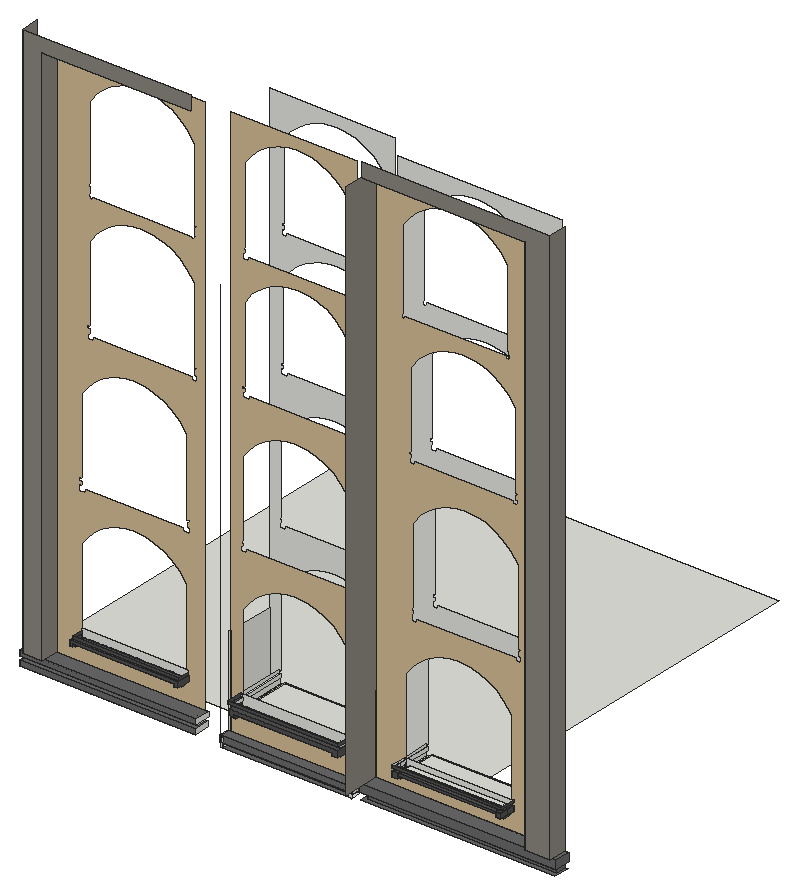
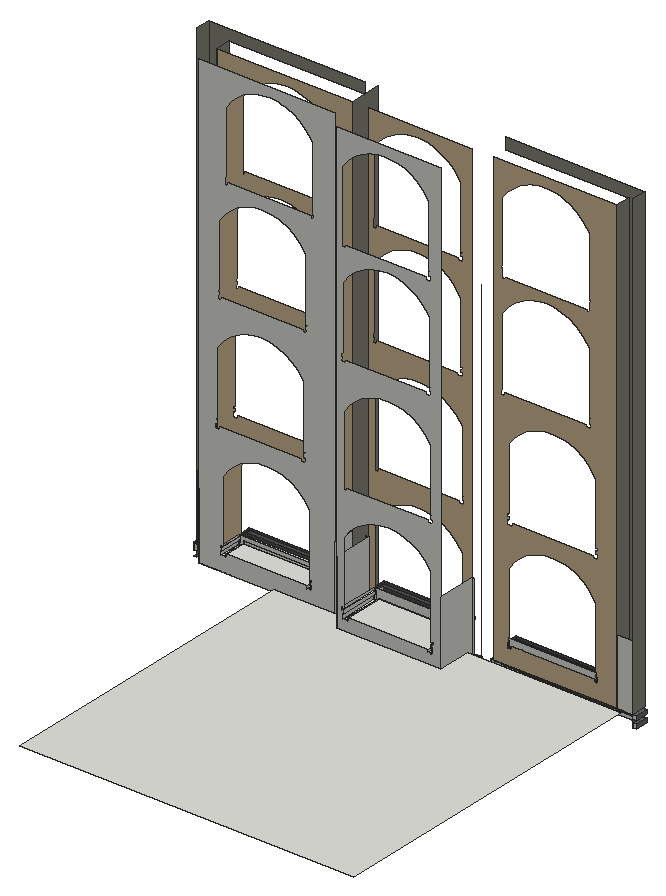
# SketchUp Ruby script. Lengths in inches.
U = 1.inch
M = Sketchup.active_model
def pt(a) = Geom::Point3d.new(a.map { |v| v * U })
def face(e, loops, mat)
  f = e.add_face(loops[0].map { |a| pt(a) })
  loops[1..].each { |l| e.add_face(l.map { |a| pt(a) }).erase! }
  f.material = f.back_material = mat if mat
  f
end
# faces: each face lists its corners as indices into pts; further lists are holes
def faces(e, pts, list, mat = nil) = list.each { |f| face(e, (f[0].is_a?(Array) ? f : [f]).map { |l| l.map { |i| pts[i] } }, mat) }
# xy, xz, yz: faces in a plane at the given z, y or x. An outline is a flat list of corners, or four numbers for a rectangle; further outlines are holes
def ring(l) = l.size == 4 ? [[l[0], l[1]], [l[2], l[1]], [l[2], l[3]], [l[0], l[3]]] : l.each_slice(2).to_a
def flat(e, list, mat, &to3) = list.each { |f| face(e, (f[0].is_a?(Array) ? f : [f]).map { |l| ring(l).map { |u, v| to3.(u, v) } }, mat) }
def xy(e, z, list, mat = nil) = flat(e, list, mat) { |x, y| [x, y, z] }
def xz(e, y, list, mat = nil) = flat(e, list, mat) { |x, z| [x, y, z] }
def yz(e, x, list, mat = nil) = flat(e, list, mat) { |y, z| [x, y, z] }
def lines(e, pts, list) = list.each { |a, b| e.add_line(pt(pts[a]), pt(pts[b])) }
# prism: a flat outline (further loops are holes) pulled along v
def prism(e, loops, v, mat = nil)
  f = face(e, loops, mat); d = Geom::Vector3d.new(v.map { |x| x * U })
  f.pushpull(f.normal.samedirection?(d) ? d.length : -d.length)
end
def box(e, o, s, mat = nil) = prism(e, [[o, [o[0] + s[0], o[1], o[2]], [o[0] + s[0], o[1] + s[1], o[2]], [o[0], o[1] + s[1], o[2]]]], [0, 0, s[2]], mat)
def at(x, y, z, deg = 0) = Geom::Transformation.translation(pt([x, y, z])) * Geom::Transformation.rotation(ORIGIN, Z_AXIS, deg.degrees)
def axes(o, x, y, z) = Geom::Transformation.new([*x, 0, *y, 0, *z, 0, *pt(o).to_a, 1])
def part(name) = M.definitions.add(name)
# library, detail: a bought-in or finely detailed component or shape, given as its bounding box
def library(name, o, s) = part(name).tap { |d| box(d.entities, o, s) }
def detail(e, o, s) = box(e.add_group.entities, o, s)
def put(e, d, t, mat = nil) = e.add_instance(d, t).tap { |i| i.material = mat if mat }
def group(e, t, mat = nil) = e.add_group.tap { |g| g.transformation = t; g.material = mat if mat }.entities
root = M.entities
M.materials.add("[0134_DimGray]").color = [105, 105, 105]
M.materials.add("[0135_DarkGray]").color = [81, 81, 81]
M.materials.add("[Formica Beige]").color = [211, 187, 149]
M.materials.add("[Formica Graystone]").color = [137, 134, 124]
M.materials.add("[Formica Graystone]1").color = [149, 146, 135]
xy(root,125.87,[[224.47,37.6875,226.6,49.6875],[226.6,37.6875,227.04,43.6875],[370.55,37.6875,370.74,43.6875],[370.74,37.6875,374.55,49.6875],[226.6,43.6875,227.04,49.6875],
  [370.55,43.6875,370.74,49.6875],[224.47,49.6875,226.6,107.5]])
xy(root,125.87,[[227.04,37.6875,370.55,43.6875]],"[0134_DimGray]")
xy(root,130.6875,[[223.66,37.6875,223.66,49.6875,226.6,49.6875,226.6,43.6875,370.74,43.6875,370.74,49.6875,375.3,49.6875,375.3,37.6875]],"[0134_DimGray]")
xy(root,131.98,[[389.32,31.6875,611.75,31.6875,611.75,49.6875,608.5,49.6875,608.5,37.6875,392.7,37.6875,392.7,49.6875,389.32,49.6875]],"[0134_DimGray]")
xy(root,132.82,[[0,31.6875,0,49.6875,4.9375,49.6875,4.9375,37.6875,197.35,37.6875,197.35,49.6875,200.6,49.6875,200.6,31.6875]],"[0134_DimGray]")
xy(root,137.74,[[227.04,49.6875,370.55,104.375]])
xy(root,137.74,[[223.66,37.6875,375.3,49.6875]],"[0134_DimGray]")
xy(root,138.5625,[[0,31.6875,200.6,31.6875,200.6,49.6875,197.35,49.6875,197.35,37.6875,4.9375,37.6875,4.9375,49.6875,0,49.6875]],"[0134_DimGray]")
xy(root,139.38,[[387.45,31.6875,387.45,49.6875,392.7,49.6875,392.7,37.6875,608.5,37.6875,608.5,49.6875,612.75,49.6875,612.75,31.6875]],"[0134_DimGray]")
xy(root,143.01,[[0,31.6875,0,49.6875,4.9375,49.6875,4.9375,37.6875,197.35,37.6875,197.35,49.6875,200.97,49.6875,200.97,31.6875]],"[0134_DimGray]")
xy(root,148.75,[[4.9375,31.6875,27.68,49.6875],[387.45,31.6875,392.7,49.6875],[392.7,49.6875,475.9375,80.4375],[475.9375,49.6875,580.01,80.4375]])
xy(root,148.75,[[4.9375,28.6875,27.68,31.6875],[0,31.6875,4.9375,49.6875],[27.68,31.6875,200.97,49.6875],[392.7,31.6875,580.01,49.6875],[580.01,31.6875,612.75,49.6875]],"[0134_DimGray]")
xy(root,149.0625,[[580.01,28.6875,608.5,49.6875]],"[Formica Graystone]1")
xy(root,151.875,[[13.9375,58.6875,475.9375,520.6875]])
xy(root,163.35,[[238.57,34.7,244.63,40.6875]],"[0135_DarkGray]")
xy(root,164.72,[[356.01,37.12,362.82,42.6]],"[0135_DarkGray]")
xy(root,165.85,[[238.57,49.6875,240.45,104.375],[240.45,49.6875,244.63,104.375],[356.01,49.6875,360.89,104.375],[360.89,49.6875,362.82,104.375]])
xy(root,165.85,[[238.57,31.6875,244.63,34.7],[356.01,31.6875,362.82,37.12],[238.57,40.6875,244.63,49.6875],[356.01,42.6,362.82,49.6875]],"[0135_DarkGray]")
xy(root,166.35,[[425.07,35.9375,431.66,40.6875]],"[0135_DarkGray]")
xy(root,167.35,[[543.375,36.53,549.7,42.4375]],"[0135_DarkGray]")
xy(root,168.72,[[425.07,35.9375,426.95,40.6875],[426.95,35.9375,431.66,40.6875],[543.375,36.53,548.14,40.6875],[548.14,36.53,549.7,40.6875],[543.375,40.6875,548.14,42.4375],
  [548.14,40.6875,549.7,42.4375],[425.07,49.6875,426.95,80.4375],[426.95,49.6875,431.66,80.4375],[543.375,49.6875,548.14,80.4375],[548.14,49.6875,549.7,80.4375]])
xy(root,168.72,[[425.07,31.6875,426.95,35.9375],[426.95,31.6875,431.66,35.9375],[543.375,31.6875,548.14,36.53],[548.14,31.6875,549.7,36.53],[425.07,40.6875,426.95,49.6875],
  [426.95,40.6875,431.66,49.6875],[543.375,42.4375,548.14,49.6875],[548.14,42.4375,549.7,49.6875]],"[0135_DarkGray]")
xy(root,168.85,[[244.63,49.6875,356.01,104.375]])
xy(root,168.85,[[244.63,31.6875,356.01,49.6875]],"[0135_DarkGray]")
xy(root,169.47,[[54.45,39.33,58.06,43.45]],"[0135_DarkGray]")
xy(root,169.78,[[173.8125,39.99,177.95,43.12]],"[0135_DarkGray]")
xy(root,171.22,[[54.45,34.6875,58.06,39.33],[173.8125,34.6875,177.95,39.99],[173.8125,43.12,177.95,49.6875],[54.45,43.45,58.06,49.6875]],"[0135_DarkGray]")
xy(root,171.72,[[431.66,49.6875,543.375,80.4375]])
xy(root,171.72,[[431.66,31.6875,543.375,49.6875]],"[0135_DarkGray]")
xy(root,172.92,[[238.57,49.6875,240.45,104.375],[360.89,49.6875,362.82,104.375]])
xy(root,172.92,[[238.57,31.6875,362.82,31.6875,362.82,49.6875,360.89,49.6875,360.89,37.6875,240.45,37.6875,240.45,49.6875,238.57,49.6875]],"[0135_DarkGray]")
xy(root,174.22,[[58.06,34.6875,173.8125,49.6875]],"[0135_DarkGray]")
xy(root,174.33,[[431.66,37.6875,543.375,49.6875],[425.07,49.6875,426.95,80.4375],[548.14,49.6875,549.7,80.4375]])
xy(root,174.33,[[425.07,31.6875,426.95,40.6875],[426.95,31.6875,431.66,37.6875],[431.66,31.6875,543.375,37.6875],[543.375,31.6875,548.14,37.6875],[548.14,31.6875,549.7,40.6875],
  [425.07,40.6875,426.95,49.6875],[548.14,40.6875,549.7,49.6875]],"[0135_DarkGray]")
xy(root,176.99,[[237.76,49.6875,240.45,104.375],[360.89,49.6875,363.26,104.375]])
xy(root,176.99,[[237.76,31.6875,237.76,49.6875,240.45,49.6875,240.45,37.6875,360.89,37.6875,360.89,49.6875,363.26,49.6875,363.26,31.6875]],"[0135_DarkGray]")
xy(root,177.23,[[54.45,34.6875,177.95,34.6875,177.95,49.6875,176.89,49.6875,176.89,37.6875,55.95,37.6875,55.95,49.6875,54.45,49.6875]],"[0135_DarkGray]")
xy(root,178.09,[[425.2,40.6875,426.95,49.6875],[425.2,49.6875,426.95,80.4375],[548.14,49.6875,549.95,80.4375]])
xy(root,178.09,[[425.2,31.6875,426.95,40.6875],[426.95,31.6875,548.14,37.6875],[548.14,31.6875,549.95,40.6875],[548.14,40.6875,549.95,49.6875]],"[0135_DarkGray]")
xz(root,28.6875,[[4.9375,148.75,27.68,148.75,27.68,772.09,197.35,772.09,197.35,787.6875,4.9375,787.6875],[580.01,149.0625,608.5,149.0625,608.5,787.6875,392.7,787.6875,392.7,772.09,580.01,772.09]],"[Formica Graystone]")
xz(root,31.6875,[[0,132.82,200.6,138.5625],[387.45,139.38,612.75,148.75],[0,143.01,200.97,148.75]],"[0134_DimGray]")
xz(root,31.6875,[[238.57,165.85,244.63,165.85,244.63,168.85,356.01,168.85,356.01,165.85,362.82,165.85,362.82,172.92,238.57,172.92],[425.07,168.72,431.66,174.33],[543.375,168.72,549.7,174.33],[431.66,171.72,543.375,174.33],[237.76,176.99,363.26,180.28],
  [425.2,178.09,549.95,180.28]],"[0135_DarkGray]")
xz(root,34.6875,[[54.45,171.22,58.06,171.22,58.06,174.22,173.8125,174.22,173.8125,171.22,177.95,171.22,177.95,177.23,54.45,177.23]],"[0135_DarkGray]")
xz(root,34.7,[[238.57,163.35,244.63,165.85]],"[0135_DarkGray]")
xz(root,35.9375,[[425.07,166.35,431.66,168.72]],"[0135_DarkGray]")
xz(root,36.53,[[543.375,167.35,549.7,168.72]],"[0135_DarkGray]")
xz(root,37.12,[[356.01,164.72,362.82,165.85]],"[0135_DarkGray]")
xz(root,37.6875,[[224.47,125.87,226.6,130.6875],[226.6,125.87,227.04,130.6875],[370.74,125.87,374.55,130.6875],[223.66,130.6875,224.47,137.74],[224.47,130.6875,226.6,137.74],
  [226.6,130.6875,227.04,137.74],[370.55,130.6875,370.74,137.74],[370.74,130.6875,374.55,137.74],[374.55,130.6875,375.3,137.74],[4.9375,132.82,197.35,138.5625]])
xz(root,37.6875,[[227.04,130.6875,370.55,137.74],[392.7,131.98,608.5,139.38],[4.9375,138.5625,197.35,143.01]],"[0134_DimGray]")
xz(root,37.6875,[[240.45,172.92,360.89,176.99],[426.95,174.33,548.14,178.09],[55.95,177.23,176.89,180.23]],"[0135_DarkGray]")
xz(root,39.33,[[54.45,169.47,58.06,171.22]],"[0135_DarkGray]")
xz(root,39.99,[[173.8125,169.78,177.95,171.22]],"[0135_DarkGray]")
xz(root,40.6875,[[238.57,163.35,244.63,165.85],[425.07,166.35,431.66,168.72]])
xz(root,42.4375,[[543.375,167.35,549.7,168.72]])
xz(root,42.6,[[356.01,164.72,362.82,165.85]])
xz(root,43.12,[[173.8125,169.78,177.95,171.22]])
xz(root,43.45,[[54.45,169.47,58.06,171.22]])
xz(root,43.6875,[[226.6,125.87,370.74,130.6875]],"[0134_DimGray]")
xz(root,49.6875,[[224.47,125.87,226.6,130.6875],[226.6,125.87,227.04,130.6875],[370.55,125.87,370.74,130.6875],[370.74,125.87,374.55,130.6875],[223.66,130.6875,224.47,137.74],
  [224.47,130.6875,226.6,137.74],[226.6,130.6875,227.04,137.74],[370.55,130.6875,370.74,137.74],[370.74,130.6875,374.55,137.74],[374.55,130.6875,375.3,137.74],
  [0,132.82,4.9375,138.5625],[197.35,132.82,200.6,138.5625],[224.47,137.74,226.6,240],[226.6,137.74,227.04,240],[370.55,137.74,370.74,240],
  [370.74,137.74,374.55,240],[387.45,139.38,392.7,148.75],[608.5,139.38,612.75,148.75],[0,143.01,4.9375,148.75],[197.35,143.01,200.97,148.75],
  [4.9375,148.75,27.68,240],[580.01,148.75,608.5,149.0625],[580.01,149.0625,608.5,240],[238.57,165.85,240.45,172.92],[240.45,165.85,244.63,165.85,244.63,168.85,356.01,168.85,356.01,165.85,360.89,165.85,360.89,180.28,240.45,180.28],
  [360.89,165.85,362.82,172.92],[425.07,168.72,426.95,174.33],[426.95,168.72,426.95,180.28,548.14,180.28,548.14,168.72,543.375,168.72,543.375,174.33,431.66,174.33,431.66,168.72],[548.14,168.72,549.7,174.33],[54.45,171.22,55.95,177.23],
  [55.95,171.22,58.06,171.22,58.06,174.22,173.8125,174.22,173.8125,171.22,176.89,171.22,176.89,183.1,55.95,183.1],[176.89,171.22,177.95,177.23],[431.66,171.72,543.375,174.33]])
xz(root,49.6875,[[[227.04,137.74,370.55,772.09],[238.57,165.85,238.57,172.92,240.45,172.92,240.45,176.99,237.76,176.99,237.76,180.28,240.45,180.28,240.45,266.7,249.375,278.3,257.84,286.17,267.5,292.53,278.07,297.2,289.27,300.05,300.79,301.01,312.3125,300.05,323.51,297.2,334.09,292.53,343.74,286.17,352.21,278.3,361.14,266.7,361.14,180.28,363.26,180.28,363.26,176.99,360.89,176.99,360.89,172.92,362.82,172.92,362.82,165.85,356.01,165.85,356.01,168.85,244.63,168.85,244.63,165.85],[240.7,626.53,240.7,633.11,242.82,633.11,242.82,636.68,240.7,636.68,240.7,638.72,242.82,638.72,242.82,725.13,251.75,736.74,260.22,744.61,269.87,750.96,276.84,754.04,280.45,755.63,286.31,757.13,291.65,758.49,303.17,759.45,314.6875,758.49,320.02,757.13,325.89,755.63,329.5,754.04,336.46,750.96,346.11,744.61,354.58,736.74,363.51,725.13,363.51,638.72,363.89,638.72,363.89,626.53,358.47,626.53,358.47,629.53,246.92,629.53,246.92,626.53],[240.07,484.28,240.07,490.18,242.14,490.18,242.14,493.07,239.45,493.07,239.45,495.66,242.14,495.66,242.14,582.07,251.0625,593.68,259.53,601.54,269.18,607.9,276.15,610.98,279.76,612.57,290.96,615.43,302.48,616.39,314,615.43,325.2,612.57,328.81,610.98,335.77,607.9,345.43,601.54,353.9,593.68,362.82,582.07,362.82,495.66,364.64,495.66,364.64,490.18,363.14,490.18,363.14,487.28,364.76,487.28,364.76,484.28,358.5,484.28,358.5,487.28,247.74,487.28,247.74,484.28],[238.45,326.47,238.45,332.04,240.45,332.04,240.45,334.61,238.64,334.61,238.64,336.85,240.45,336.85,240.45,423.26,249.375,434.86,257.84,442.73,267.5,449.09,278.07,453.76,289.27,456.61,300.79,457.57,312.3125,456.61,323.51,453.76,334.09,449.09,343.74,442.73,352.21,434.86,361.14,423.26,361.14,336.85,361.32,336.85,361.32,326.47,356.5625,326.47,356.5625,329.47,245.25,329.47,245.25,326.47]],[[27.68,148.75,197.35,772.09],[53.26,323.16,53.26,329.79,55.95,329.79,55.95,333.42,52.82,333.42,52.82,336.85,55.95,336.85,55.95,423.26,64.875,434.86,73.34,442.73,83,449.09,93.57,453.76,104.77,456.61,116.29,457.57,127.8125,456.61,139.01,453.76,149.59,449.09,159.24,442.73,167.71,434.86,176.64,423.26,176.64,336.85,179.26,336.85,179.26,333.42,176.89,333.42,176.89,329.79,179.82,329.79,179.82,323.16,171.09,323.16,171.09,326.16,60.625,326.16,60.625,323.16],[62.57,481.97,62.57,487.85,64.89,487.85,64.89,493.17,62.39,493.17,62.39,495.66,64.89,495.66,64.89,582.07,73.8125,593.68,82.28,601.54,91.93,607.9,98.9,610.98,102.51,612.57,113.71,615.43,125.23,616.39,136.75,615.43,147.95,612.57,151.56,610.98,158.52,607.9,168.18,601.54,176.65,593.68,185.57,582.07,185.57,495.66,187.14,495.66,187.14,493.17,185.82,493.17,185.82,487.85,187.51,487.85,187.51,481.97,181.99,481.97,181.99,484.97,69.5625,484.97,69.5625,481.97],[64.89,625.91,64.89,627.98,63.89,627.98,63.89,630.86,64.89,630.86,64.89,638.17,63.64,638.17,63.64,641.05,64.89,641.05,64.89,725.13,73.8125,736.74,82.28,744.61,91.93,750.96,98.9,754.04,102.51,755.63,108.37,757.13,113.71,758.49,125.23,759.45,136.75,758.49,142.09,757.13,147.95,755.63,151.56,754.04,158.52,750.96,168.18,744.61,176.65,736.74,185.57,725.13,185.57,641.05,187.39,641.05,187.39,638.17,185.57,638.17,185.57,630.86,186.64,630.86,186.64,627.98,185.57,627.98,185.57,626.47,180.6,626.47,180.6,627.97,69.04,627.97,69.04,625.91],[54.45,171.22,54.45,177.23,55.95,177.23,55.95,180.23,54.57,180.23,54.57,183.1,55.95,183.1,55.95,269.51,64.875,281.11,73.34,288.98,83,295.34,93.57,300.01,104.77,302.86,116.29,303.82,127.8125,302.86,139.01,300.01,149.59,295.34,159.24,288.98,167.71,281.11,176.64,269.51,176.64,183.1,177.76,183.1,177.76,180.23,176.89,180.23,176.89,177.23,177.95,177.23,177.95,171.22,173.8125,171.22,173.8125,174.22,58.06,174.22,58.06,171.22]],[[392.7,148.75,580.01,772.09],[433.26,323.47,433.26,330.36,434.7,330.36,434.7,334.01,433.14,334.01,433.14,336.85,434.7,336.85,434.7,423.26,443.625,434.86,452.09,442.73,461.75,449.09,472.32,453.76,483.52,456.61,495.04,457.57,506.5625,456.61,517.76,453.76,528.34,449.09,537.99,442.73,546.46,434.86,555.39,423.26,555.39,336.85,557.64,336.85,557.64,334.01,556.01,334.01,556.01,330.36,558.14,330.36,558.14,323.47,551.95,323.47,551.95,326.47,438.96,326.47,438.96,323.47],[425.07,168.72,425.07,174.33,426.95,174.33,426.95,178.09,425.2,178.09,425.2,180.28,426.95,180.28,426.95,266.7,435.875,278.3,444.34,286.17,454,292.53,464.57,297.2,475.77,300.05,487.29,301.01,498.8125,300.05,510.01,297.2,520.59,292.53,530.24,286.17,538.71,278.3,547.64,266.7,547.64,180.28,549.95,180.28,549.95,178.09,548.14,178.09,548.14,174.33,549.7,174.33,549.7,168.72,543.375,168.72,543.375,171.72,431.66,171.72,431.66,168.72],[430.82,484.03,430.82,489.3125,432.14,489.3125,432.14,492.99,430.01,492.99,430.01,495.66,432.14,495.66,432.14,582.07,441.0625,593.68,449.53,601.54,459.18,607.9,466.15,610.98,469.76,612.57,480.96,615.43,492.48,616.39,504,615.43,515.2,612.57,518.81,610.98,525.77,607.9,535.43,601.54,543.9,593.68,552.82,582.07,552.82,495.66,554.64,495.66,554.64,492.99,552.7,492.99,552.7,489.3125,554.39,489.3125,554.39,484.03,549.38,484.03,549.38,487.03,437.43,487.03,437.43,484.03],[421.76,629.35,421.76,634.06,423.07,634.06,423.07,725.13,432,736.74,440.47,744.61,450.12,750.96,457.09,754.04,460.7,755.63,466.56,757.13,471.9,758.49,483.42,759.45,494.9375,758.49,500.27,757.13,506.14,755.63,509.75,754.04,516.71,750.96,526.36,744.61,534.83,736.74,543.76,725.13,543.76,638.72,544.82,638.72,544.82,637.05,543.95,637.05,543.95,634.06,544.95,634.06,544.95,629.35,541.16,629.35,541.16,632.35,425.87,632.35,425.87,629.35]]],"[Formica Beige]")
xz(root,80.4375,[[[392.7,148.75,580.01,772.09],[433.26,323.47,438.96,323.47,438.96,326.47,551.95,326.47,551.95,323.47,558.14,323.47,558.14,330.36,556.01,330.36,556.01,334.01,557.64,334.01,557.64,336.85,555.39,336.85,555.39,423.26,546.46,434.86,537.99,442.73,528.34,449.09,517.76,453.76,506.5625,456.61,495.04,457.57,483.52,456.61,472.32,453.76,461.75,449.09,452.09,442.73,443.625,434.86,434.7,423.26,434.7,336.85,433.14,336.85,433.14,334.01,434.7,334.01,434.7,330.36,433.26,330.36],[425.07,168.72,431.66,168.72,431.66,171.72,543.375,171.72,543.375,168.72,549.7,168.72,549.7,174.33,548.14,174.33,548.14,178.09,549.95,178.09,549.95,180.28,547.64,180.28,547.64,266.7,538.71,278.3,530.24,286.17,520.59,292.53,510.01,297.2,498.8125,300.05,487.29,301.01,475.77,300.05,464.57,297.2,454,292.53,444.34,286.17,435.875,278.3,426.95,266.7,426.95,180.28,425.2,180.28,425.2,178.09,426.95,178.09,426.95,174.33,425.07,174.33],[430.82,484.03,437.43,484.03,437.43,487.03,549.38,487.03,549.38,484.03,554.39,484.03,554.39,489.3125,552.7,489.3125,552.7,492.99,554.64,492.99,554.64,495.66,552.82,495.66,552.82,582.07,543.9,593.68,535.43,601.54,525.77,607.9,518.81,610.98,515.2,612.57,504,615.43,492.48,616.39,480.96,615.43,469.76,612.57,466.15,610.98,459.18,607.9,449.53,601.54,441.0625,593.68,432.14,582.07,432.14,495.66,430.01,495.66,430.01,492.99,432.14,492.99,432.14,489.3125,430.82,489.3125],[421.76,629.35,425.87,629.35,425.87,632.35,541.16,632.35,541.16,629.35,544.95,629.35,544.95,634.06,543.95,634.06,543.95,637.05,544.82,637.05,544.82,638.72,543.76,638.72,543.76,725.13,534.83,736.74,526.36,744.61,516.71,750.96,509.75,754.04,506.14,755.63,500.27,757.13,494.9375,758.49,483.42,759.45,471.9,758.49,466.56,757.13,460.7,755.63,457.09,754.04,450.12,750.96,440.47,744.61,432,736.74,423.07,725.13,423.07,634.06,421.76,634.06]]])
xz(root,104.375,[[[227.04,137.74,370.55,772.09],[238.57,165.85,244.63,165.85,244.63,168.85,356.01,168.85,356.01,165.85,362.82,165.85,362.82,172.92,360.89,172.92,360.89,176.99,363.26,176.99,363.26,180.28,361.14,180.28,361.14,266.7,352.21,278.3,343.74,286.17,334.09,292.53,323.51,297.2,312.3125,300.05,300.79,301.01,289.27,300.05,278.07,297.2,267.5,292.53,257.84,286.17,249.375,278.3,240.45,266.7,240.45,180.28,237.76,180.28,237.76,176.99,240.45,176.99,240.45,172.92,238.57,172.92],[240.7,626.53,246.92,626.53,246.92,629.53,358.47,629.53,358.47,626.53,363.89,626.53,363.89,638.72,363.51,638.72,363.51,725.13,354.58,736.74,346.11,744.61,336.46,750.96,329.5,754.04,325.89,755.63,320.02,757.13,314.6875,758.49,303.17,759.45,291.65,758.49,286.31,757.13,280.45,755.63,276.84,754.04,269.87,750.96,260.22,744.61,251.75,736.74,242.82,725.13,242.82,638.72,240.7,638.72,240.7,636.68,242.82,636.68,242.82,633.11,240.7,633.11],[240.07,484.28,247.74,484.28,247.74,487.28,358.5,487.28,358.5,484.28,364.76,484.28,364.76,487.28,363.14,487.28,363.14,490.18,364.64,490.18,364.64,495.66,362.82,495.66,362.82,582.07,353.9,593.68,345.43,601.54,335.77,607.9,328.81,610.98,325.2,612.57,314,615.43,302.48,616.39,290.96,615.43,279.76,612.57,276.15,610.98,269.18,607.9,259.53,601.54,251.0625,593.68,242.14,582.07,242.14,495.66,239.45,495.66,239.45,493.07,242.14,493.07,242.14,490.18,240.07,490.18],[238.45,326.47,245.25,326.47,245.25,329.47,356.5625,329.47,356.5625,326.47,361.32,326.47,361.32,336.85,361.14,336.85,361.14,423.26,352.21,434.86,343.74,442.73,334.09,449.09,323.51,453.76,312.3125,456.61,300.79,457.57,289.27,456.61,278.07,453.76,267.5,449.09,257.84,442.73,249.375,434.86,240.45,423.26,240.45,336.85,238.64,336.85,238.64,334.61,240.45,334.61,240.45,332.04,238.45,332.04]]])
yz(root,0,[[31.6875,132.82,49.6875,138.5625],[31.6875,143.01,49.6875,148.75]],"[0134_DimGray]")
yz(root,4.9375,[[37.6875,132.82,49.6875,138.5625]])
yz(root,4.9375,[[37.6875,138.5625,49.6875,143.01]],"[0134_DimGray]")
yz(root,4.9375,[[28.6875,148.75,49.6875,787.6875]],"[Formica Graystone]")
yz(root,27.68,[[28.6875,148.75,49.6875,772.09]],"[Formica Graystone]")
yz(root,54.45,[[39.33,169.47,39.33,171.22,34.6875,171.22,34.6875,177.23,49.6875,177.23,49.6875,171.22,43.45,171.22,43.45,169.47]],"[0135_DarkGray]")
yz(root,55.95,[[37.6875,177.23,49.6875,180.23]],"[0135_DarkGray]")
yz(root,58.06,[[39.33,169.47,43.45,169.47,43.45,171.22,49.6875,171.22,49.6875,174.22,34.6875,174.22,34.6875,171.22,39.33,171.22]],"[0135_DarkGray]")
yz(root,173.8125,[[39.99,169.78,39.99,171.22,34.6875,171.22,34.6875,174.22,49.6875,174.22,49.6875,171.22,43.12,171.22,43.12,169.78]],"[0135_DarkGray]")
yz(root,176.89,[[37.6875,177.23,49.6875,180.23]],"[0135_DarkGray]")
yz(root,177.95,[[39.99,169.78,43.12,169.78,43.12,171.22,49.6875,171.22,49.6875,177.23,34.6875,177.23,34.6875,171.22,39.99,171.22]],"[0135_DarkGray]")
yz(root,197.35,[[37.6875,132.82,49.6875,138.5625],[37.6875,138.5625,49.6875,143.01]])
yz(root,200.6,[[31.6875,132.82,49.6875,138.5625]])
yz(root,200.97,[[31.6875,143.01,49.6875,148.75]])
yz(root,223.66,[[37.6875,130.6875,49.6875,137.74]])
yz(root,226.6,[[43.6875,125.87,49.6875,130.6875]])
yz(root,227.04,[[49.6875,137.74,104.375,240]])
yz(root,237.76,[[49.6875,176.99,104.375,180.28]])
yz(root,237.76,[[31.6875,176.99,49.6875,180.28]],"[0135_DarkGray]")
yz(root,238.57,[[49.6875,165.85,104.375,172.92]])
yz(root,238.57,[[34.7,163.35,34.7,165.85,31.6875,165.85,31.6875,172.92,49.6875,172.92,49.6875,165.85,40.6875,165.85,40.6875,163.35]],"[0135_DarkGray]")
yz(root,240.45,[[37.6875,172.92,49.6875,176.99],[49.6875,172.92,104.375,176.99]])
yz(root,244.63,[[49.6875,165.85,104.375,168.85]])
yz(root,244.63,[[34.7,163.35,40.6875,163.35,40.6875,165.85,49.6875,165.85,49.6875,168.85,31.6875,168.85,31.6875,165.85,34.7,165.85]],"[0135_DarkGray]")
yz(root,356.01,[[49.6875,165.85,104.375,168.85]])
yz(root,356.01,[[37.12,164.72,37.12,165.85,31.6875,165.85,31.6875,168.85,49.6875,168.85,49.6875,165.85,42.6,165.85,42.6,164.72]],"[0135_DarkGray]")
yz(root,360.89,[[37.6875,172.92,49.6875,176.99],[49.6875,172.92,104.375,176.99]])
yz(root,362.82,[[49.6875,165.85,104.375,172.92]])
yz(root,362.82,[[37.12,164.72,42.6,164.72,42.6,165.85,49.6875,165.85,49.6875,172.92,31.6875,172.92,31.6875,165.85,37.12,165.85]],"[0135_DarkGray]")
yz(root,363.26,[[49.6875,176.99,104.375,180.28]])
yz(root,363.26,[[31.6875,176.99,49.6875,180.28]],"[0135_DarkGray]")
yz(root,370.55,[[49.6875,137.74,104.375,240]])
yz(root,370.74,[[43.6875,125.87,49.6875,130.6875]])
yz(root,375.3,[[37.6875,130.6875,49.6875,137.74]])
yz(root,387.45,[[31.6875,139.38,49.6875,148.75]])
yz(root,392.7,[[37.6875,131.98,49.6875,139.38],[49.6875,148.75,80.4375,240]])
yz(root,392.7,[[6,148.75,49.6875,772.09]],"[Formica Graystone]")
yz(root,425.07,[[35.9375,166.35,40.6875,168.72],[31.6875,168.72,40.6875,174.33],[40.6875,168.72,49.6875,174.33],[49.6875,168.72,80.4375,174.33]])
yz(root,425.2,[[31.6875,178.09,40.6875,180.28],[40.6875,178.09,49.6875,180.28],[49.6875,178.09,80.4375,180.28]])
yz(root,426.95,[[37.6875,174.33,40.6875,178.09],[40.6875,174.33,49.6875,178.09],[49.6875,174.33,80.4375,178.09]])
yz(root,431.66,[[49.6875,168.72,80.4375,171.72],[31.6875,171.72,40.6875,174.33],[40.6875,171.72,49.6875,174.33]])
yz(root,431.66,[[35.9375,166.35,40.6875,168.72],[31.6875,168.72,40.6875,171.72],[40.6875,168.72,49.6875,171.72]],"[0135_DarkGray]")
yz(root,543.375,[[49.6875,168.72,80.4375,171.72],[31.6875,171.72,40.6875,174.33],[40.6875,171.72,49.6875,174.33]])
yz(root,543.375,[[36.53,167.35,42.4375,168.72],[31.6875,168.72,40.6875,171.72],[40.6875,168.72,49.6875,171.72]],"[0135_DarkGray]")
yz(root,548.14,[[49.6875,174.33,80.4375,178.09]])
yz(root,548.14,[[37.6875,174.33,40.6875,178.09],[40.6875,174.33,49.6875,178.09]],"[0135_DarkGray]")
yz(root,549.7,[[49.6875,168.72,80.4375,174.33]])
yz(root,549.7,[[36.53,167.35,42.4375,168.72],[31.6875,168.72,40.6875,174.33],[40.6875,168.72,49.6875,174.33]],"[0135_DarkGray]")
yz(root,549.95,[[49.6875,178.09,80.4375,180.28]])
yz(root,549.95,[[31.6875,178.09,40.6875,180.28],[40.6875,178.09,49.6875,180.28]],"[0135_DarkGray]")
yz(root,580.01,[[40.6875,148.75,49.6875,149.0625],[49.6875,148.75,80.4375,149.0625],[49.6875,149.0625,80.4375,240]])
yz(root,580.01,[[28.6875,149.0625,49.6875,772.09]],"[Formica Graystone]")
yz(root,608.5,[[37.6875,131.98,49.6875,139.38]],"[0134_DimGray]")
yz(root,608.5,[[28.6875,149.0625,49.6875,787.6875]],"[Formica Graystone]")
yz(root,612.75,[[31.6875,139.38,49.6875,148.75]],"[0134_DimGray]")
p = [[370.74,43.6875,130.6875],[370.74,43.6875,137.74],[608.5,37.6875,139.38],[608.5,37.6875,148.75],[197.35,37.6875,143.01],[197.35,37.6875,148.75],
  [224.47,37.6875,137.74],[224.47,37.6875,600],[55.95,37.6875,174.22],[55.95,37.6875,177.23],[176.89,37.6875,177.23],[176.89,37.6875,174.22],
  [360.89,37.6875,180.28],[360.89,37.6875,176.99],[240.45,37.6875,176.99],[240.45,37.6875,180.28],[360.89,37.6875,172.92],[360.89,37.6875,168.85],
  [240.45,37.6875,168.85],[240.45,37.6875,172.92],[426.95,37.6875,171.72],[426.95,37.6875,174.33],[548.14,37.6875,180.28],[548.14,37.6875,178.09],
  [426.95,37.6875,178.09],[426.95,37.6875,180.28]]
lines(root,p,[[0,1],[2,3],[4,5],[6,7],[8,9],[10,11],[12,13],[14,15],[16,17],[18,19],[20,21],[22,23],
  [24,25]])
